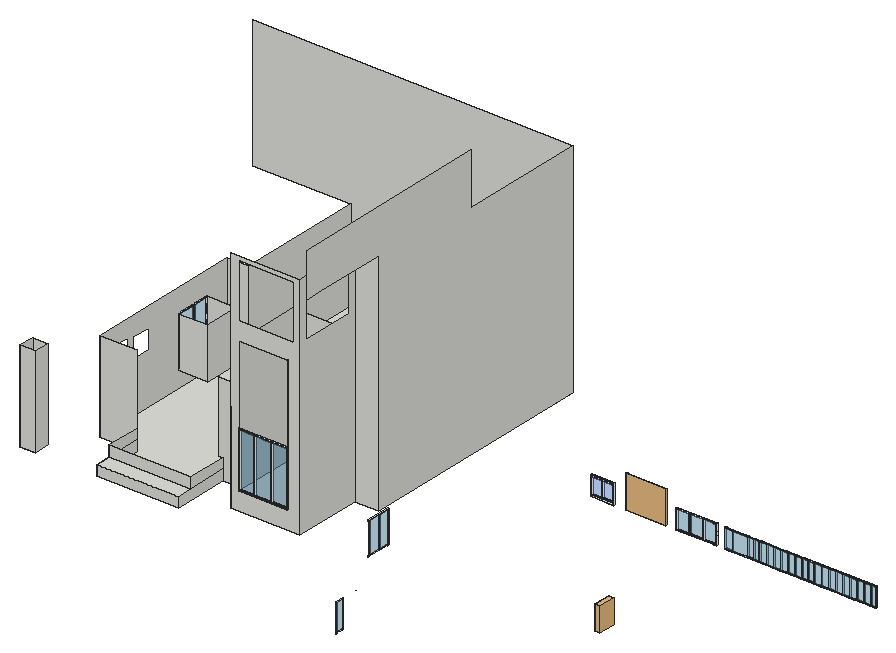
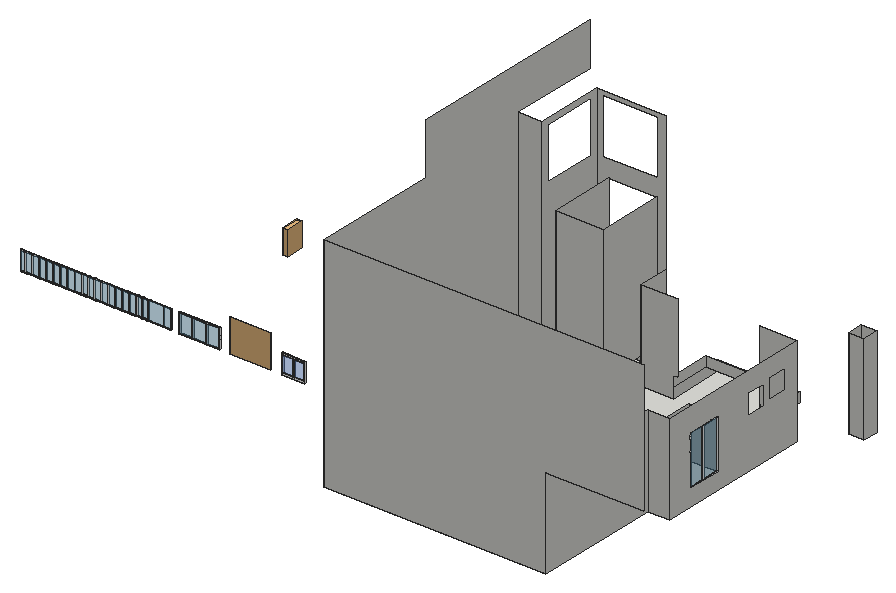
# SketchUp Ruby script. Lengths in inches.
U = 1.inch
M = Sketchup.active_model
def pt(a) = Geom::Point3d.new(a.map { |v| v * U })
def face(e, loops, mat)
  f = e.add_face(loops[0].map { |a| pt(a) })
  loops[1..].each { |l| e.add_face(l.map { |a| pt(a) }).erase! }
  f.material = f.back_material = mat if mat
  f
end
# faces: each face lists its corners as indices into pts; further lists are holes
def faces(e, pts, list, mat = nil) = list.each { |f| face(e, (f[0].is_a?(Array) ? f : [f]).map { |l| l.map { |i| pts[i] } }, mat) }
# xy, xz, yz: faces in a plane at the given z, y or x. An outline is a flat list of corners, or four numbers for a rectangle; further outlines are holes
def ring(l) = l.size == 4 ? [[l[0], l[1]], [l[2], l[1]], [l[2], l[3]], [l[0], l[3]]] : l.each_slice(2).to_a
def flat(e, list, mat, &to3) = list.each { |f| face(e, (f[0].is_a?(Array) ? f : [f]).map { |l| ring(l).map { |u, v| to3.(u, v) } }, mat) }
def xy(e, z, list, mat = nil) = flat(e, list, mat) { |x, y| [x, y, z] }
def xz(e, y, list, mat = nil) = flat(e, list, mat) { |x, z| [x, y, z] }
def yz(e, x, list, mat = nil) = flat(e, list, mat) { |y, z| [x, y, z] }
def lines(e, pts, list) = list.each { |a, b| e.add_line(pt(pts[a]), pt(pts[b])) }
# prism: a flat outline (further loops are holes) pulled along v
def prism(e, loops, v, mat = nil)
  f = face(e, loops, mat); d = Geom::Vector3d.new(v.map { |x| x * U })
  f.pushpull(f.normal.samedirection?(d) ? d.length : -d.length)
end
def box(e, o, s, mat = nil) = prism(e, [[o, [o[0] + s[0], o[1], o[2]], [o[0] + s[0], o[1] + s[1], o[2]], [o[0], o[1] + s[1], o[2]]]], [0, 0, s[2]], mat)
def at(x, y, z, deg = 0) = Geom::Transformation.translation(pt([x, y, z])) * Geom::Transformation.rotation(ORIGIN, Z_AXIS, deg.degrees)
def axes(o, x, y, z) = Geom::Transformation.new([*x, 0, *y, 0, *z, 0, *pt(o).to_a, 1])
def part(name) = M.definitions.add(name)
# library, detail: a bought-in or finely detailed component or shape, given as its bounding box
def library(name, o, s) = part(name).tap { |d| box(d.entities, o, s) }
def detail(e, o, s) = box(e.add_group.entities, o, s)
def put(e, d, t, mat = nil) = e.add_instance(d, t).tap { |i| i.material = mat if mat }
def group(e, t, mat = nil) = e.add_group.tap { |g| g.transformation = t; g.material = mat if mat }.entities
root = M.entities
M.materials.add("Translucent_Glass_Blue1").color = [100, 149, 237]
M.materials["Translucent_Glass_Blue1"].alpha = 0.5
M.materials.add("[Color_000]").color = [255, 255, 255]
M.materials.add("[Color_A23]1").color = [66, 26, 26]
M.materials.add("[Jade]").color = [77, 143, 110]
M.materials.add("[Translucent_Glass_Blue]1").color = [87, 149, 181]
M.materials["[Translucent_Glass_Blue]1"].alpha = 0.5
c1 = part("Group\#4")
xy(c1.entities,0,[[21.26,0,22.68,1.42]],"[Color_000]")
xy(c1.entities,1.42,[[0,0,1.42,0.57],[1.42,0,21.26,1.42]],"[Color_000]")
xy(c1.entities,72.28,[[0,0,1.42,0.57],[1.42,0,21.26,1.42]],"[Color_000]")
xy(c1.entities,73.7,[[0,0,21.26,1.42],[21.26,0,22.68,1.42]],"[Color_000]")
xz(c1.entities,0,[[0,0,21.26,1.42],[21.26,0,22.68,73.7],[0,72.28,21.26,73.7]],"[Color_000]")
xz(c1.entities,0.57,[[0,1.42,1.42,72.28]],"[Color_000]")
xz(c1.entities,1.42,[[21.26,0,22.68,73.7]],"[Color_000]")
xz(c1.entities,1.42,[[1.42,1.42,21.26,72.28]],"[Translucent_Glass_Blue]1")
yz(c1.entities,0,[[0.57,1.42,1.42,72.28]],"[Color_000]")
yz(c1.entities,1.42,[[0.57,1.42,1.42,72.28]],"[Color_000]")
yz(c1.entities,21.26,[[0,0,1.42,1.42],[0,1.42,1.42,72.28]],"[Color_000]")
yz(c1.entities,22.68,[[0,0,1.42,27.92],[0,27.92,1.42,41.1],[0,41.1,1.42,73.7]],"[Color_000]")
c2 = part("Series SC7600 3/4 Hour Fire Rated Steel Self Closing Horizon")
xy(c2.entities,0,[[-43.42,-60.88,-3.84,-6.07],[1.5,-60.88,42.9375,-5.86]],"Translucent_Glass_Blue1")
g1 = group(c2.entities,at(-48,-66.92,4.1875))
xy(g1,-4.1875,[[[0,0,96,66.92],[2.49,4.05,93.43,62.75]]])
xy(g1,-0.875,[[2.49,4.05,44.17,4.05,44.17,6.04,4.58,6.04,4.58,60.85,44.17,60.85,44.17,62.75,2.49,62.75],[[47.96,4.05,93.43,62.75],[49.5,6.04,90.9375,61.0625]]])
xy(g1,0,[[[0,0,96,66.92],[2.49,4.05,93.43,62.75]],[44.17,4.05,47.96,62.75]])
xz(g1,0,[[0,-4.1875,96,0]])
xz(g1,4.05,[[2.49,-4.1875,44.17,-0.875],[44.17,-4.1875,47.96,0],[47.96,-4.1875,93.43,-0.875],[2.49,-0.875,44.17,0],[47.96,-0.875,93.43,0]])
xz(g1,6.04,[[4.58,-4.1875,44.17,-0.875],[49.5,-4.1875,90.9375,-0.875]])
xz(g1,60.85,[[4.58,-4.1875,44.16,-0.875],[44.16,-4.1875,44.17,-0.875]])
xz(g1,61.0625,[[49.5,-4.1875,86.89,-0.875],[86.89,-4.1875,90.9375,-0.875]])
xz(g1,62.75,[[2.49,-4.1875,44.17,-0.875],[44.17,-4.1875,47.96,0],[47.96,-4.1875,93.43,-0.875],[2.49,-0.875,44.17,0],[47.96,-0.875,93.43,0]])
xz(g1,66.92,[[0,-4.1875,96,0]])
yz(g1,0,[[0,-4.1875,66.92,0]])
yz(g1,2.49,[[4.05,-4.1875,62.75,-0.875],[4.05,-0.875,62.75,0]])
yz(g1,4.58,[[6.04,-4.1875,60.85,-0.875]])
yz(g1,44.17,[[6.04,-4.1875,60.85,0],[4.05,-0.875,6.04,0],[60.85,-0.875,62.75,0]])
yz(g1,47.96,[[4.05,-0.875,62.75,0]])
yz(g1,49.5,[[6.04,-4.1875,7.3,-0.875],[7.3,-4.1875,61.0625,-0.875]])
yz(g1,90.9375,[[6.04,-4.1875,61.0625,-0.875]])
yz(g1,93.43,[[4.05,-4.1875,62.75,-0.875],[4.05,-0.875,62.75,0]])
yz(g1,96,[[0,-4.1875,66.92,0]])
c3 = library("Bowed window grille",[0,0,0],[13.04,44.69,63.99])
c4 = part("Group\#3")
xy(c4.entities,0,[[0,0,2.14,2.21]],"[Color_000]")
xy(c4.entities,1.67,[[2.14,0,29.96,2.21],[29.96,0,32.1,0.88],[32.1,0,64.19,2.21],[64.19,0,66.33,0.88]],"[Color_000]")
xy(c4.entities,84.95,[[2.14,0,29.96,2.21],[29.96,0,32.1,0.88],[32.1,0,64.19,2.21],[64.19,0,66.33,0.88]],"[Color_000]")
xy(c4.entities,86.61,[[0,0,66.33,2.21]],"[Color_000]")
xz(c4.entities,0,[[0,0,0,86.61,66.33,86.61,66.33,84.95,2.14,84.95,2.14,0],[2.14,0,66.33,1.67]],"[Color_000]")
xz(c4.entities,0.88,[[29.96,1.67,32.1,84.95],[64.19,1.67,66.33,84.95]],"[Color_000]")
xz(c4.entities,2.21,[[2.14,1.67,29.96,84.95],[32.1,1.67,64.19,84.95]],"[Translucent_Glass_Blue]1")
yz(c4.entities,0,[[0,0,2.21,32.8125],[0,32.8125,2.21,48.3],[0,48.3,2.21,86.61]],"[Color_000]")
yz(c4.entities,2.14,[[0,1.67,2.21,84.95]],"[Color_000]")
yz(c4.entities,29.96,[[0.88,1.67,2.21,84.95]],"[Color_000]")
yz(c4.entities,32.1,[[0.88,1.67,2.21,84.95]],"[Color_000]")
yz(c4.entities,64.19,[[0.88,1.67,2.21,84.95]],"[Color_000]")
yz(c4.entities,66.33,[[0.88,1.67,2.21,84.95]],"[Color_000]")
c5 = library("Group\#2",[0,0,0],[106.3,86.61,1.97])
c6 = part("Group\#66")
xy(c6.entities,0,[[8858.27,0,9055.12,10236.22]],"[Color_000]")
xy(c6.entities,0,[[196.85,196.85,2755.91,10039.37],[2952.76,196.85,5905.51,10039.37],[6102.36,196.85,8858.27,10039.37]],"[Translucent_Glass_Blue]1")
xy(c6.entities,118.11,[[2755.91,196.85,2952.76,10039.37],[5905.51,196.85,6102.36,10039.37]],"[Color_000]")
xy(c6.entities,196.85,[[0,0,0,10236.22,8858.27,10236.22,8858.27,10039.37,196.85,10039.37,196.85,0],[196.85,0,8858.27,196.85],[8858.27,0,9055.12,10236.22]],"[Color_000]")
xz(c6.entities,0,[[0,0,196.85,196.85],[196.85,0,8858.27,196.85],[8858.27,0,9055.12,196.85]],"[Color_000]")
xz(c6.entities,196.85,[[196.85,0,2755.91,196.85],[2952.76,0,5905.51,196.85],[6102.36,0,8858.27,196.85],[2755.91,118.11,2952.76,196.85],[5905.51,118.11,6102.36,196.85]],"[Color_000]")
xz(c6.entities,10039.37,[[196.85,0,2755.91,196.85],[2952.76,0,5905.51,196.85],[6102.36,0,8858.27,196.85],[2755.91,118.11,2952.76,196.85],[5905.51,118.11,6102.36,196.85]],"[Color_000]")
xz(c6.entities,10236.22,[[0,0,8858.27,196.85],[8858.27,0,9055.12,196.85]],"[Color_000]")
yz(c6.entities,0,[[0,0,3877.95,196.85],[3877.95,0,5708.66,196.85],[5708.66,0,10236.22,196.85]],"[Color_000]")
yz(c6.entities,196.85,[[196.85,0,10039.37,196.85]],"[Color_000]")
yz(c6.entities,2755.91,[[196.85,0,10039.37,118.11]],"[Color_000]")
yz(c6.entities,2952.76,[[196.85,0,10039.37,118.11]],"[Color_000]")
yz(c6.entities,5905.51,[[196.85,0,10039.37,118.11]],"[Color_000]")
yz(c6.entities,6102.36,[[196.85,0,10039.37,118.11]],"[Color_000]")
yz(c6.entities,8858.27,[[0,0,196.85,196.85],[196.85,0,10039.37,196.85]],"[Color_000]")
yz(c6.entities,9055.12,[[0,0,3877.95,196.85],[3877.95,0,5708.66,196.85],[5708.66,0,10236.22,196.85]],"[Color_000]")
xy(root,0,[[98.56,244.91,139.12,285.48],[298.73,246.52,298.73,378.52,200.3125,378.52,200.3125,798.52,258.9375,798.52,258.9375,1134.21,845.125,1134.21,845.125,493.58,782.0625,493.58,782.0625,313.58,600,313.58,600,394.71,514.54,394.71,514.54,246.52]])
xy(root,27.34,[[298.73,246.52,514.54,288.02]])
xy(root,43.74,[[200.3125,638.47,277.875,731.65]])
xy(root,50.56,[[622.16,313.58,748.91,489.89]])
xz(root,244.91,[[98.56,0,139.12,240]])
xz(root,246.52,[[298.73,0,514.54,27.34]])
xz(root,285.48,[[98.56,0,139.12,240]])
xz(root,288.02,[[298.73,27.34,514.54,54.6875]])
xz(root,313.58,[[[600,0,782.0625,604.41],[622.16,50.56,748.91,404.37],[619.66,449.51,764.48,594.33]]])
xz(root,378.52,[[200.3125,0,298.73,240]])
xz(root,394.71,[[514.54,0,600,0,600,240,502.61,240,502.61,54.6875,514.54,54.6875]])
xz(root,489.89,[[622.16,50.56,748.91,404.37]])
xz(root,493.58,[[782.0625,0,845.125,604.875]])
xz(root,638.47,[[200.3125,43.74,277.875,177.99]])
xz(root,731.65,[[200.3125,43.74,277.875,177.99]])
xz(root,798.52,[[200.3125,0,258.9375,240]])
xz(root,1134.21,[[258.9375,0,258.9375,240,0,240,0,584.21,845.125,584.21,845.125,0]])
yz(root,98.56,[[244.91,0,285.48,240]])
yz(root,139.12,[[244.91,0,285.48,240]])
yz(root,200.3125,[[[378.52,0,798.52,240],[638.47,43.74,731.65,177.99],[488.22,134.84,540.72,187.34],[420.82,142.375,472.44,194]]])
yz(root,258.9375,[[798.52,0,1134.21,240]])
yz(root,277.875,[[638.47,43.74,731.65,177.99]])
yz(root,298.73,[[246.52,0,378.52,27.34],[288.02,27.34,378.52,54.6875]])
yz(root,514.54,[[246.52,0,394.71,27.34],[288.02,27.34,394.71,54.6875]])
yz(root,600,[[313.58,0,394.71,240]])
yz(root,622.16,[[313.58,50.56,489.89,404.37]])
yz(root,748.91,[[313.58,50.56,489.89,404.37]])
yz(root,782.0625,[[[313.58,0,493.58,0,493.58,604.875,313.58,604.41],[331.61,453.66,475.8,589.16]]])
yz(root,845.125,[[493.58,0,1134.21,0,1134.21,584.21,798.52,584.21,798.52,720,258.52,720,258.52,604.41,313.58,604.41,493.58,604.875]])
p = [[1020.3,201.12,2.52],[1018.89,201.12,2.52]]
lines(root,p,[[0,1]])
put(root,c1,at(1018.89,158.6,-71.18,-90))
put(root,c2,axes([1177.79,819.92,51.18],[0.65617,0,0],[0,0,0.76476],[0,-0.71939,0]),"[Color_000]")
put(root,c3,at(1508.0625,379.8,0))
put(root,c4,at(948.42,396.48,0,-90))
g2 = group(root,at(1373.45,819.34,51.48),"[Color_A23]1")
xy(g2,-51.18,[[0,-3.58,104.14,0],[104.14,-3.58,106.46,0]],"[Color_000]")
xy(g2,-50.2,[[2.3125,-3.58,32.4,0],[32.4,-3.58,34.71,-2.15],[34.71,-3.58,69.43,0],[69.43,-3.58,71.74,-2.15],[71.74,-3.58,104.14,0]],"[Color_000]")
xy(g2,-0.98,[[2.3125,-3.58,32.4,0],[32.4,-3.58,34.71,-2.15],[34.71,-3.58,69.43,0],[69.43,-3.58,71.74,-2.15],[71.74,-3.58,104.14,0]],"[Color_000]")
xy(g2,0,[[0,-3.58,2.3125,0],[2.3125,-3.58,104.14,0],[104.14,-3.58,106.46,0]],"[Color_000]")
xz(g2,-3.58,[[0,-51.18,104.14,-51.18,104.14,-50.2,2.3125,-50.2,2.3125,0,0,0],[104.14,-51.18,106.46,0],[2.3125,-0.98,104.14,0]],"[Color_000]")
xz(g2,-2.15,[[32.4,-50.2,34.71,-0.98],[69.43,-50.2,71.74,-0.98]],"[Color_000]")
xz(g2,0,[[104.14,-51.18,106.46,0]],"[Color_000]")
xz(g2,0,[[2.3125,-50.2,32.4,-0.98],[34.71,-50.2,69.43,-0.98],[71.74,-50.2,104.14,-0.98]],"[Translucent_Glass_Blue]1")
yz(g2,0,[[-3.58,-51.18,0,-28.54],[-3.58,-28.54,0,-19.39],[-3.58,-19.39,0,0]],"[Color_000]")
yz(g2,2.3125,[[-3.58,-50.2,0,-0.98]],"[Color_000]")
yz(g2,32.4,[[-2.15,-50.2,0,-0.98]],"[Color_000]")
yz(g2,34.71,[[-2.15,-50.2,0,-0.98]],"[Color_000]")
yz(g2,69.43,[[-2.15,-50.2,0,-0.98]],"[Color_000]")
yz(g2,71.74,[[-2.15,-50.2,0,-0.98]],"[Color_000]")
yz(g2,104.14,[[-3.58,-50.2,0,-0.98],[-3.58,-0.98,0,0]],"[Color_000]")
yz(g2,106.46,[[-3.58,-51.18,0,-28.54],[-3.58,-28.54,0,-19.39],[-3.58,-19.39,0,0]],"[Color_000]")
g3 = group(root,at(1501.56,815.76,51.48),"[Color_000]")
xy(g3,-51.18,[[0,0,346.46,1.18],[346.46,0,399.61,1.18]])
xy(g3,-50.2,[[0.98,0,20.67,1.18],[21.65,0,38.39,1.18],[38.39,0,60.04,1.18],[93.5,0,111.22,1.18],[112.2,0,129.92,1.18],
  [130.91,0,148.62,1.18],[149.61,0,167.32,1.18],[168.31,0,186.02,1.18],[187.01,0,187.99,1.18],[187.99,0,204.72,1.18],
  [205.71,0,221.46,0.98],[221.46,0,237.2,0.98],[238.1875,0,255.91,1.18],[256.89,0,274.61,1.18],[275.59,0,293.31,1.18],
  [294.29,0,312.01,1.18],[312.99,0,330.71,1.18],[331.69,0,347.44,1.18],[347.44,0,349.41,1.18],[350.39,0,368.11,1.18],
  [369.09,0,386.8125,1.18],[387.8,0,398.62,1.18],[61.02,0.98,76.77,1.18],[76.77,0.98,92.52,1.18],[205.71,0.98,221.46,1.18],
  [221.46,0.98,237.2,1.18]])
xy(g3,-49.21,[[62.01,0,75.79,0.98],[77.76,0,91.54,0.98],[206.69,0,220.47,0.98],[222.44,0,236.22,0.98]])
xy(g3,-0.98,[[0.98,0,20.67,1.18],[21.65,0,60.04,1.18],[62.01,0,75.79,0.98],[77.76,0,91.54,0.98],[93.5,0,111.22,1.18],
  [112.2,0,129.92,1.18],[130.91,0,148.62,1.18],[149.61,0,167.32,1.18],[168.31,0,186.02,1.18],[187.01,0,204.72,1.18],
  [206.69,0,220.47,0.98],[222.44,0,235.79,0.98],[235.79,0,236.22,0.98],[238.1875,0,255.91,1.18],[256.89,0,274.61,1.18],
  [274.61,0,275.59,1.18],[275.59,0,293.31,1.18],[294.29,0,312.01,1.18],[312.99,0,330.71,1.18],[331.69,0,349.41,1.18],
  [350.39,0,368.11,1.18],[369.09,0,386.8125,1.18],[387.8,0,398.62,1.18]])
xy(g3,0,[[0,0,61.02,1.18],[61.02,0,76.77,0.98],[76.77,0,92.52,0.98],[92.52,0,205.71,1.18],[205.71,0,221.46,0.98],
  [221.46,0,221.46,0.98,237.2,0.98,237.2,1.18,399.61,1.18,399.61,0]])
xz(g3,0,[[[0,-51.18,399.61,-51.18,399.61,0,237.2,0,237.2,-50.2,205.71,-50.2,205.71,0,92.52,0,92.52,-50.2,61.02,-50.2,61.02,0,0,0],[21.65,-50.2,60.04,-0.98],[256.89,-50.2,256.89,-0.98,293.31,-0.98,293.31,-50.2,275.59,-50.2,275.59,-0.98,274.61,-0.98,274.61,-50.2],[0.98,-50.2,20.67,-0.98],[187.01,-50.2,204.72,-0.98],[112.2,-50.2,129.92,-0.98],[238.1875,-50.2,255.91,-0.98],[331.69,-50.2,349.41,-0.98],[93.5,-50.2,111.22,-0.98],[312.99,-50.2,330.71,-0.98],[294.29,-50.2,312.01,-0.98],[369.09,-50.2,386.8125,-0.98],[350.39,-50.2,368.11,-0.98],[130.91,-50.2,148.62,-0.98],[149.61,-50.2,167.32,-0.98],[168.31,-50.2,186.02,-0.98],[387.8,-50.2,398.62,-0.98]]])
xz(g3,0,[[0.98,-50.2,20.67,-0.98],[21.65,-50.2,60.04,-0.98],[93.5,-50.2,111.22,-0.98],[112.2,-50.2,129.92,-0.98],[130.91,-50.2,148.62,-0.98],
  [149.61,-50.2,167.32,-0.98],[168.31,-50.2,186.02,-0.98],[187.01,-50.2,204.72,-0.98],[238.1875,-50.2,255.91,-0.98],[256.89,-50.2,274.61,-0.98],
  [275.59,-50.2,293.31,-0.98],[294.29,-50.2,312.01,-0.98],[312.99,-50.2,330.71,-0.98],[331.69,-50.2,349.41,-0.98],[350.39,-50.2,368.11,-0.98],
  [369.09,-50.2,386.8125,-0.98],[387.8,-50.2,398.62,-0.98],[62.01,-49.21,75.79,-0.98],[77.76,-49.21,91.54,-0.98],[206.69,-49.21,220.47,-0.98],
  [222.44,-49.21,236.22,-0.98]],"[Translucent_Glass_Blue]1")
xz(g3,0.98,[[[61.02,-50.2,76.77,0],[62.01,-49.21,75.79,-0.98]],[[76.77,-50.2,92.52,0],[77.76,-49.21,91.54,-0.98]],[[205.71,-50.2,221.46,0],[206.69,-49.21,220.47,-0.98]],[[221.46,-50.2,237.2,0],[222.44,-49.21,236.22,-0.98]]])
xz(g3,1.18,[[[0,-51.18,399.61,-51.18,399.61,0,237.2,0,237.2,-50.2,205.71,-50.2,205.71,0,92.52,0,92.52,-50.2,61.02,-50.2,61.02,0,0,0],[21.65,-50.2,60.04,-0.98],[256.89,-50.2,256.89,-0.98,293.31,-0.98,293.31,-50.2,275.59,-50.2,275.59,-0.98,274.61,-0.98,274.61,-50.2],[0.98,-50.2,20.67,-0.98],[187.01,-50.2,204.72,-0.98],[112.2,-50.2,129.92,-0.98],[238.1875,-50.2,255.91,-0.98],[331.69,-50.2,349.41,-0.98],[93.5,-50.2,111.22,-0.98],[312.99,-50.2,330.71,-0.98],[294.29,-50.2,312.01,-0.98],[369.09,-50.2,386.8125,-0.98],[350.39,-50.2,368.11,-0.98],[130.91,-50.2,148.62,-0.98],[149.61,-50.2,167.32,-0.98],[168.31,-50.2,186.02,-0.98],[387.8,-50.2,398.62,-0.98]]])
yz(g3,0,[[0,-51.18,1.18,0]])
yz(g3,0.98,[[0,-50.2,1.18,-0.98]])
yz(g3,20.67,[[0,-50.2,1.18,-0.98]])
yz(g3,21.65,[[0,-50.2,1.18,-0.98]])
yz(g3,60.04,[[0,-50.2,1.18,-0.98]])
yz(g3,61.02,[[0.98,-50.2,1.18,0]])
yz(g3,62.01,[[0,-49.21,0.98,-0.98]])
yz(g3,75.79,[[0,-49.21,0.98,-0.98]])
yz(g3,77.76,[[0,-49.21,0.98,-0.98]])
yz(g3,91.54,[[0,-49.21,0.98,-0.98]])
yz(g3,92.52,[[0.98,-50.2,1.18,-19.39],[0.98,-19.39,1.18,0]])
yz(g3,93.5,[[0,-50.2,1.18,-0.98]])
yz(g3,111.22,[[0,-50.2,1.18,-0.98]])
yz(g3,112.2,[[0,-50.2,1.18,-0.98]])
yz(g3,129.92,[[0,-50.2,1.18,-0.98]])
yz(g3,130.91,[[0,-50.2,1.18,-0.98]])
yz(g3,148.62,[[0,-50.2,1.18,-0.98]])
yz(g3,149.61,[[0,-50.2,1.18,-0.98]])
yz(g3,167.32,[[0,-50.2,1.18,-0.98]])
yz(g3,168.31,[[0,-50.2,1.18,-0.98]])
yz(g3,186.02,[[0,-50.2,1.18,-0.98]])
yz(g3,187.01,[[0,-50.2,1.18,-0.98]])
yz(g3,204.72,[[0,-50.2,1.18,-0.98]])
yz(g3,205.71,[[0,-50.2,0.98,-19.39],[0.98,-50.2,1.18,-19.39],[0,-19.39,0.98,0],[0.98,-19.39,1.18,0]])
yz(g3,206.69,[[0,-49.21,0.98,-0.98]])
yz(g3,220.47,[[0,-49.21,0.98,-0.98]])
yz(g3,222.44,[[0,-49.21,0.98,-0.98]])
yz(g3,236.22,[[0,-49.21,0.98,-0.98]])
yz(g3,237.2,[[0,-50.2,0.98,-0.98],[0.98,-50.2,1.18,-0.98],[0.98,-0.98,1.18,0]])
yz(g3,238.1875,[[0,-50.2,1.18,-0.98]])
yz(g3,255.91,[[0,-50.2,1.18,-0.98]])
yz(g3,256.89,[[0,-50.2,1.18,-0.98]])
yz(g3,274.61,[[0,-50.2,1.18,-0.98]])
yz(g3,275.59,[[0,-50.2,1.18,-0.98]])
yz(g3,293.31,[[0,-50.2,1.18,-0.98]])
yz(g3,294.29,[[0,-50.2,1.18,-0.98]])
yz(g3,312.01,[[0,-50.2,1.18,-0.98]])
yz(g3,312.99,[[0,-50.2,1.18,-0.98]])
yz(g3,330.71,[[0,-50.2,1.18,-0.98]])
yz(g3,331.69,[[0,-50.2,1.18,-0.98]])
yz(g3,349.41,[[0,-50.2,1.18,-0.98]])
yz(g3,350.39,[[0,-50.2,1.18,-0.98]])
yz(g3,368.11,[[0,-50.2,1.18,-0.98]])
yz(g3,369.09,[[0,-50.2,1.18,-0.98]])
yz(g3,386.8125,[[0,-50.2,1.18,-0.98]])
yz(g3,387.8,[[0,-50.2,1.18,-0.98]])
yz(g3,398.62,[[0,-50.2,1.18,-0.98]])
yz(g3,399.61,[[0,-51.18,1.18,0]])
p = [[76.77,0,-50.2],[76.77,0.98,-50.2],[92.52,0,-50.2],[92.52,0.98,-50.2],[92.52,0,-19.39],[92.52,0.98,-19.39],
  [61.02,0,-50.2],[61.02,0.98,-50.2],[130.91,0,-0.98],[129.92,0,-0.98],[149.61,0,-0.98],[148.62,0,-0.98]]
lines(g3,p,[[0,1],[2,3],[4,5],[6,7],[8,9],[10,11]])
put(root,c5,axes([1238.88,819.1,0.3],[1,0,0],[0,0,1],[0,-1,0]))
put(root,c4,axes([200.3125,731.65,43.74],[0,-1.39,0],[1,0,0],[0,0,1.54998]))
put(root,c6,axes([620.74,315,49.14],[0.0144,0,0],[0,0,0.0144],[0,-0.0144,0]),"[Jade]")
